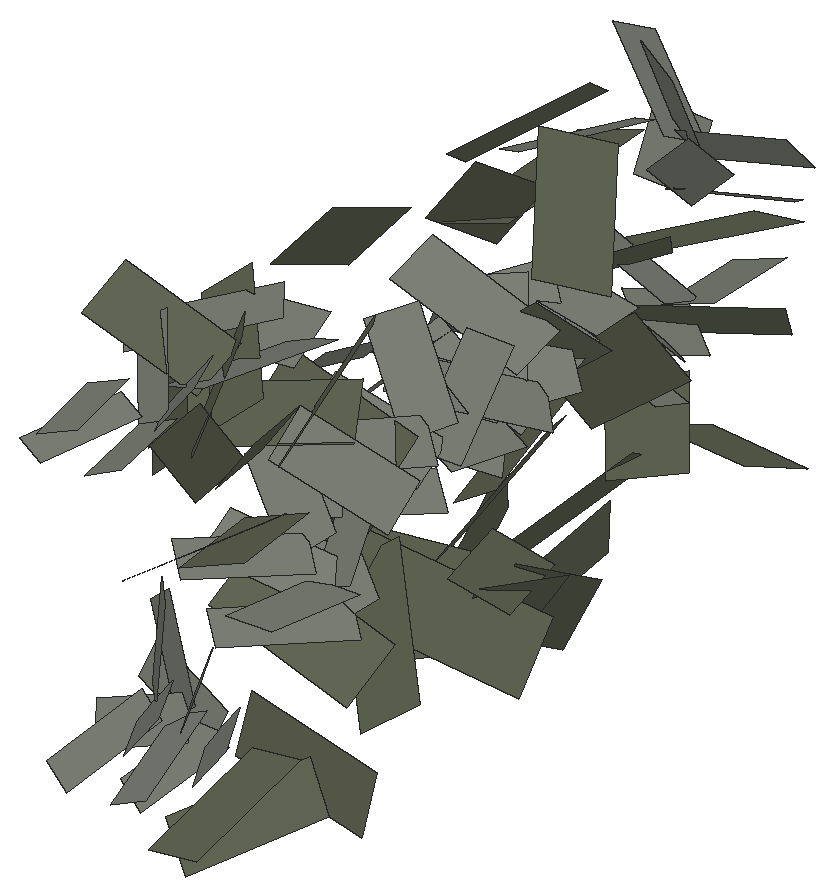
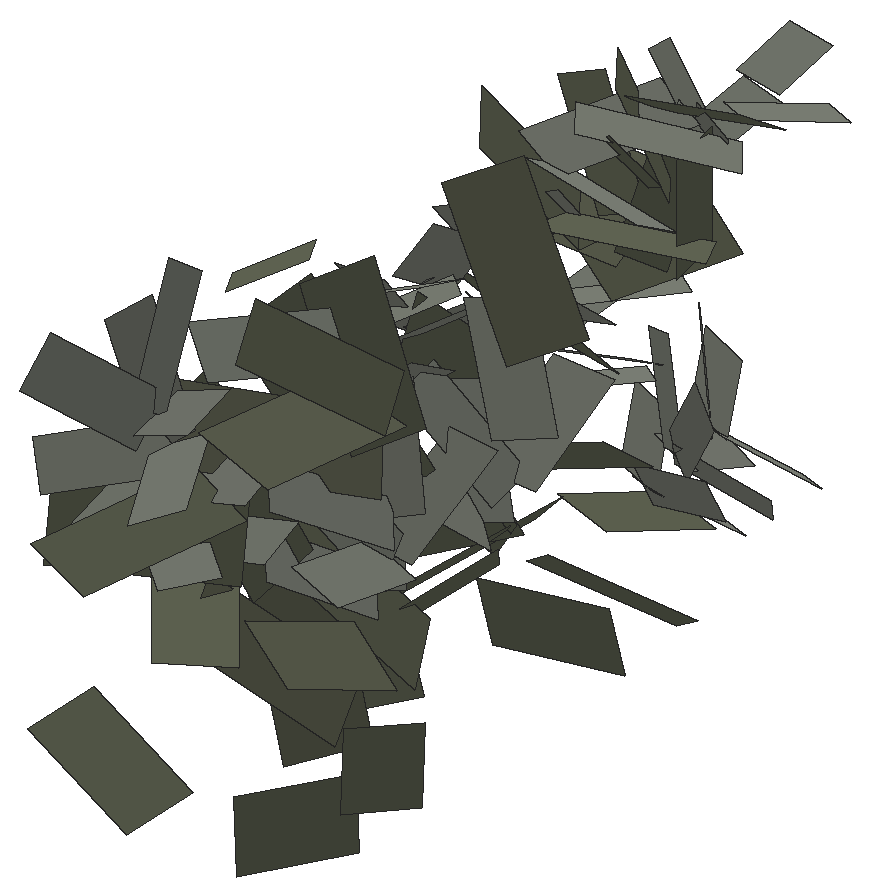
# SketchUp Ruby script. Lengths in inches.
U = 1.inch
M = Sketchup.active_model
def pt(a) = Geom::Point3d.new(a.map { |v| v * U })
def face(e, loops, mat)
  f = e.add_face(loops[0].map { |a| pt(a) })
  loops[1..].each { |l| e.add_face(l.map { |a| pt(a) }).erase! }
  f.material = f.back_material = mat if mat
  f
end
# faces: each face lists its corners as indices into pts; further lists are holes
def faces(e, pts, list, mat = nil) = list.each { |f| face(e, (f[0].is_a?(Array) ? f : [f]).map { |l| l.map { |i| pts[i] } }, mat) }
# xy, xz, yz: faces in a plane at the given z, y or x. An outline is a flat list of corners, or four numbers for a rectangle; further outlines are holes
def ring(l) = l.size == 4 ? [[l[0], l[1]], [l[2], l[1]], [l[2], l[3]], [l[0], l[3]]] : l.each_slice(2).to_a
def flat(e, list, mat, &to3) = list.each { |f| face(e, (f[0].is_a?(Array) ? f : [f]).map { |l| ring(l).map { |u, v| to3.(u, v) } }, mat) }
def xy(e, z, list, mat = nil) = flat(e, list, mat) { |x, y| [x, y, z] }
def xz(e, y, list, mat = nil) = flat(e, list, mat) { |x, z| [x, y, z] }
def yz(e, x, list, mat = nil) = flat(e, list, mat) { |y, z| [x, y, z] }
def lines(e, pts, list) = list.each { |a, b| e.add_line(pt(pts[a]), pt(pts[b])) }
# prism: a flat outline (further loops are holes) pulled along v
def prism(e, loops, v, mat = nil)
  f = face(e, loops, mat); d = Geom::Vector3d.new(v.map { |x| x * U })
  f.pushpull(f.normal.samedirection?(d) ? d.length : -d.length)
end
def box(e, o, s, mat = nil) = prism(e, [[o, [o[0] + s[0], o[1], o[2]], [o[0] + s[0], o[1] + s[1], o[2]], [o[0], o[1] + s[1], o[2]]]], [0, 0, s[2]], mat)
def at(x, y, z, deg = 0) = Geom::Transformation.translation(pt([x, y, z])) * Geom::Transformation.rotation(ORIGIN, Z_AXIS, deg.degrees)
def axes(o, x, y, z) = Geom::Transformation.new([*x, 0, *y, 0, *z, 0, *pt(o).to_a, 1])
def part(name) = M.definitions.add(name)
# library, detail: a bought-in or finely detailed component or shape, given as its bounding box
def library(name, o, s) = part(name).tap { |d| box(d.entities, o, s) }
def detail(e, o, s) = box(e.add_group.entities, o, s)
def put(e, d, t, mat = nil) = e.add_instance(d, t).tap { |i| i.material = mat if mat }
def group(e, t, mat = nil) = e.add_group.tap { |g| g.transformation = t; g.material = mat if mat }.entities
root = M.entities
M.materials.add("viburnumblaasdfas0df1w06d").color = [98, 102, 84]
M.materials.add("viburnumbladsadfasdfad0w122").color = [125, 129, 119]
c1 = part("Component\#315")
p = [[0.25,0,0],[2.05,0.01,0.35],[1.81,4.2,1.66],[0,4.19,1.3125]]
faces(c1.entities,p,[[0,1,2,3]],"viburnumbladsadfasdfad0w122")
c2 = part("viburnumblad2")
put(c2.entities,c1,axes([-19.23,-4.49,-32.18],[83.35428,0,0],[0,79.38502,0],[0,0,83.35428]))
c3 = part("Component\#314")
p = [[0.14,0,0],[2.58,0.05,0.25],[2.44,5.11,2.64],[0,5.05,2.39]]
faces(c3.entities,p,[[0,1,2,3]],"viburnumblaasdfas0df1w06d")
c4 = part("viburnumblad1\#2")
put(c4.entities,c3,axes([-37.25,6.23,19.31],[75.98784,0,0],[0,65.50676,0],[0,0,75.98784]))
put(root,c2,axes([2197.35,270.92,20.94],[0.01264,-0.00008,0.0032],[0.00017,0.01368,-0.00036],[-0.00319,0.00037,0.01263]))
put(root,c4,axes([2198.77,269.1,11.5625],[0.00484,-0.00571,0.01239],[0.00394,0.01587,0.00555],[-0.01361,0.00143,0.00513]))
put(root,c2,axes([2198.79,266.02,22.4375],[-0.0132,-0.00264,-0.00489],[0.00251,-0.01421,0.00089],[-0.00477,0.0001,0.01275]))
put(root,c4,axes([2196.78,266.52,26.34],[-0.0079,-0.01248,0.00117],[0.01398,-0.00821,0.00596],[-0.0035,0.004,0.01323]))
put(root,c2,axes([2199.56,270.78,21.55],[-0.01264,0.00008,-0.0032],[-0.00094,-0.01268,0.00342],[-0.00306,0.00351,0.01217]))
put(root,c4,axes([2198.75,256.2,24.51],[0.00244,-0.01122,0.00057],[0.00459,0.00184,0.0121],[-0.01018,-0.00173,0.00319]))
put(root,c4,axes([2196.55,273.26,27.23],[0.00379,-0.01036,0.00596],[0.01309,0.006,0.00209],[-0.00395,0.00482,0.01088]))
put(root,c4,axes([2201.18,254.32,28.69],[0.00232,0.01057,0.00577],[-0.01348,0.00407,-0.00203],[-0.00316,-0.00514,0.01068]))
put(root,c2,axes([2200.07,251.87,28.74],[-0.00892,0.00552,-0.00065],[-0.0045,-0.00791,-0.00542],[-0.00314,-0.00411,0.00807]))
put(root,c2,axes([2197.68,266.58,23.97],[-0.00718,-0.01175,-0.00394],[0.01087,-0.00815,0.00451],[-0.0058,-0.00063,0.01231]))
put(root,c2,axes([2199.07,252.96,27.46],[0.0088,0.00119,0.00472],[-0.00418,0.00904,0.00526],[-0.00322,-0.0061,0.00681]))
put(root,c4,axes([2197.79,271.04,26.21],[0.01555,-0.00131,0.00405],[0.00291,0.01735,-0.00577],[-0.00307,0.00585,0.01401]))
put(root,c2,axes([2197.32,267.03,20.32],[0.012,-0.00837,0.00311],[0.00592,0.01032,0.00492],[-0.00527,-0.00304,0.01219]))
put(root,c2,axes([2200.45,252.26,17.23],[-0.00876,0.00688,0.00103],[-0.00474,-0.00469,-0.00897],[-0.00509,-0.00746,0.00659]))
put(root,c2,axes([2200.76,253.27,16.05],[-0.0033,0.00751,0.0076],[-0.0089,0.00112,-0.00498],[-0.00448,-0.00819,0.00616]))
put(root,c2,axes([2201.45,257.38,30.71],[-0.00774,0.01238,-0.00167],[-0.01057,-0.00772,-0.00819],[-0.0074,-0.00296,0.01235]))
put(root,c2,axes([2197.1875,267.16,21.98],[0.00305,-0.01398,-0.00068],[0.01153,0.00223,0.00588],[-0.00601,-0.00193,0.01207]))
put(root,c2,axes([2197.29,272.09,22.5],[0.00854,-0.00917,0.00359],[0.00887,0.00923,0.00245],[-0.00426,0.00084,0.01229]))
put(root,c2,axes([2200.6,254.54,15.23],[0.00419,0.0043,0.00836],[-0.00938,0.00585,0.00169],[-0.00405,-0.0083,0.0063]))
put(root,c4,axes([2198.62,270.69,16.26],[0.01227,-0.00323,0.0066],[0.00379,0.01612,0.00085],[-0.00658,0.00088,0.01266]))
put(root,c2,axes([2199.51,254.22,16.22],[0.00908,-0.00221,0.00614],[-0.004,0.00655,0.00828],[-0.00518,-0.00884,0.00448]))
put(root,c2,axes([2199.6,251.82,30.03],[-0.00916,-0.00124,-0.00492],[0.00298,-0.00959,-0.00307],[-0.00406,-0.0039,0.00779]))
put(root,c2,axes([2198.85,271.8,22.94],[-0.00933,-0.00906,-0.00093],[0.0081,-0.00886,0.00508],[-0.00417,0.00306,0.01196]))
put(root,c2,axes([2201.47,257.88,28.64],[0.00099,0.01426,0.00559],[-0.01157,0.00302,-0.00566],[-0.00706,-0.00428,0.01216]))
put(root,c4,axes([2198.25,272.39,25.21],[-0.00969,-0.0086,0.00402],[0.01095,-0.00941,0.00625],[-0.00101,0.00665,0.01178]))
put(root,c4,axes([2199.29,271.49,10.8125],[0.00403,-0.00389,0.01235],[0.00756,0.01368,0.00184],[-0.01119,0.00546,0.00538]))
put(root,c4,axes([2200.93,255.43,26.7],[0.00961,0.00314,0.00694],[-0.00599,0.01265,0.00258],[-0.0056,-0.00466,0.00986]))
put(root,c2,axes([2198.74,267.11,20.93],[-0.00599,-0.01069,-0.00483],[0.01087,-0.00815,0.00451],[-0.00654,-0.00189,0.01181]))
put(root,c2,axes([2199.03,253.58,17.7],[0.00876,-0.00688,-0.00103],[0.00337,0.00275,0.0103],[-0.00608,-0.00838,0.00422]))
put(root,c2,axes([2198.37,272.06,21.01],[-0.00055,-0.01289,0.00188],[0.01116,0.00015,0.00431],[-0.00466,0.00195,0.01201]))
put(root,c2,axes([2198.32,271.62,19.47],[0.00892,-0.00957,0.00375],[0.00799,0.0083,0.0022],[-0.00426,0.00084,0.01229]))
put(root,c2,axes([2201.66,254.26,15.75],[-0.00914,0.00718,0.00108],[-0.00427,-0.00422,-0.00808],[-0.00509,-0.00746,0.00659]))
put(root,c2,axes([2201.97,277.49,28.94],[0.00139,0.01031,-0.00841],[-0.01248,0.00393,0.00276],[0.0046,0.00756,0.01003]))
put(root,c2,axes([2199.63,271.46,19.93],[-0.00812,-0.00859,-0.00204],[0.0081,-0.00886,0.00508],[-0.00515,0.00206,0.01179]))
put(root,c2,axes([2200.54,253.08,28.33],[-0.00798,-0.00075,-0.00527],[0.00298,-0.00959,-0.00307],[-0.00502,-0.00401,0.00721]))
put(root,c4,axes([2204.23,258.62,26.16],[-0.0074,0.01393,0.00333],[-0.01491,-0.00558,-0.00981],[-0.00631,-0.00654,0.01332]))
put(root,c2,axes([2198.41,273.23,29.13],[0.01161,-0.00902,0.00438],[0.00853,0.00943,-0.00297],[-0.0007,0.0056,0.01299]))
put(root,c2,axes([2201.13,276.96,27.46],[0.00973,0.00497,-0.00674],[-0.00836,0.01112,-0.00387],[0.00402,0.00678,0.0108]))
put(root,c4,axes([2200.77,256.64,24.66],[-0.00329,-0.00864,-0.00687],[0.00632,-0.00867,0.00771],[-0.00921,-0.00096,0.00528]))
put(root,c2,axes([2201.15,253.77,17.21],[-0.00908,0.00221,-0.00614],[0.00272,-0.00885,-0.00722],[-0.00599,-0.007,0.00633]))
put(root,c4,axes([2202.68,268.2,14.41],[-0.00681,0.00895,0.00759],[-0.01184,-0.01026,0.00148],[0.00579,-0.00507,0.01117]))
put(root,c4,axes([2200.12,255.04,26.2],[0.00733,-0.00886,0.00054],[0.00689,0.00642,0.00923],[-0.00652,-0.00466,0.00706]))
put(root,c2,axes([2199.67,253.81,28.29],[0.0036,-0.00945,-0.00418],[0.00778,0.00056,0.0052],[-0.00475,-0.00515,0.0067]))
put(root,c4,axes([2199.32,268.54,15.01],[0.00765,-0.01303,0.00422],[0.01267,0.01016,0.00822],[-0.00817,-0.00039,0.01254]))
put(root,c2,axes([2200.23,253.14,18.3],[-0.00409,-0.00375,-0.00971],[0.008,-0.0078,-0.00036],[-0.00665,-0.00708,0.00553]))
put(root,c4,axes([2204.46,259.39,23.27],[0.00378,0.01126,0.01091],[-0.0152,0.00977,-0.00482],[-0.0086,-0.00789,0.01113]))
put(root,c4,axes([2204.01,259.37,11.11],[0.00278,0.00293,0.01264],[-0.01346,0.00734,0.00126],[-0.00579,-0.01128,0.00389]))
put(root,c2,axes([2202.73,258.64,29.79],[-0.01142,0.0037,-0.00741],[-0.00214,-0.01514,-0.00425],[-0.0084,-0.00214,0.01187]))
put(root,c4,axes([2198.46,271.04,23.44],[0.00743,-0.01098,0.00888],[0.01612,0.00899,-0.00172],[-0.00302,0.0089,0.01251]))
put(root,c4,axes([2204.05,257.3,12.875],[-0.00836,0.0066,0.00609],[-0.00962,-0.00288,-0.01008],[-0.00344,-0.01004,0.00615]))
put(root,c2,axes([2202.46,256.5,22.25],[0.00865,0.00796,0.00491],[-0.00918,0.00854,0.00232],[-0.00184,-0.00511,0.01153]))
put(root,c2,axes([2203.73,256.68,20.85],[-0.00016,0.01206,0.00411],[-0.0133,0.00032,-0.00146],[-0.00141,-0.0041,0.01199]))
put(root,c2,axes([2200.19,254.5625,17.43],[0.0033,-0.00751,-0.0076],[0.00833,-0.00317,0.00675],[-0.00669,-0.00765,0.00466]))
put(root,c4,axes([2204.34,258.28,16.42],[0.00263,0.01141,0.00764],[-0.01577,0.00377,-0.0002],[-0.00192,-0.0074,0.01171]))
put(root,c4,axes([2203.01,256.13,23.87],[-0.00905,0.00252,-0.00817],[0.0005,-0.01365,-0.00475],[-0.00803,-0.00297,0.00749]))
put(root,c4,axes([2203.13,265.79,15.03],[-0.01009,0.00576,0.00864],[-0.00958,-0.01423,-0.00203],[0.00708,-0.00619,0.01118]))
put(root,c2,axes([2203.21,265.82,22.78],[0.00269,0.01067,0.0031],[-0.01059,0.00139,0.00439],[0.00368,-0.00386,0.01011]))
put(root,c2,axes([2204.01,256.14,22.52],[-0.00888,0.0091,0.0009],[-0.00895,-0.0084,-0.00345],[-0.00187,-0.00303,0.01224]))
put(root,c4,axes([2199.96,271.49,14.1],[0.00413,-0.01232,0.00597],[0.01417,0.00711,0.00487],[-0.00618,0.00389,0.01229]))
put(root,c2,axes([2204.13,274.625,24.71],[-0.00041,0.01136,-0.00703],[-0.01336,-0.0005,-0.00003],[-0.00029,0.00703,0.01137]))
put(root,c2,axes([2203.77,266.37,21.47],[-0.00563,0.00838,0.00295],[-0.00922,-0.00664,0.00128],[0.00288,-0.0019,0.0109]))
put(root,c4,axes([2200.15,276,24.16],[0.01373,-0.0042,0.00303],[0.00601,0.01319,-0.00893],[-0.00014,0.00827,0.01212]))
put(root,c4,axes([2201.71,260.84,19.45],[0.00372,-0.01109,0.0102],[0.00971,0.0119,0.0094],[-0.01253,0.00356,0.00844]))
put(root,c4,axes([2203.31,256.45,14.86],[-0.01158,0.00263,-0.00305],[0.00041,-0.00999,-0.01013],[-0.00401,-0.00833,0.00806]))
put(root,c2,axes([2201.36,255.22,16.76],[-0.00392,-0.0036,-0.00932],[0.00864,-0.00842,-0.00039],[-0.00665,-0.00708,0.00553]))
put(root,c2,axes([2204.02,261.58,23.2],[-0.00038,0.01114,0.00561],[-0.01176,-0.00241,0.0034],[0.00455,-0.00528,0.01006]))
put(root,c2,axes([2203.17,257.74,19.44],[0.00904,0.00831,0.00513],[-0.00826,0.00768,0.00209],[-0.00184,-0.00511,0.01153]))
put(root,c2,axes([2204.24,265.54,24.03],[-0.00577,0.00885,0.00437],[-0.00922,-0.00664,0.00128],[0.00353,-0.00288,0.01049]))
put(root,c2,axes([2203.42,277.97,28.14],[-0.01295,0.00298,0.00152],[-0.00101,-0.00935,0.0097],[0.0032,0.00918,0.00919]))
put(root,c4,axes([2200.22,269.48,20.91],[-0.01012,-0.01025,0.00891],[0.01634,-0.00922,0.0075],[0.00063,0.01164,0.0125]))
put(root,c2,axes([2204.9,273.17,21.77],[-0.00039,0.0109,-0.00675],[-0.01442,-0.00054,-0.00004],[-0.00029,0.00703,0.01137]))
put(root,c2,axes([2204.95,265.6,26.28],[0,0.01516,0.00154],[-0.01516,-0.00015,0.00148],[0.00149,-0.00153,0.01509]))
put(root,c2,axes([2204.75,257.52,19.71],[-0.00853,0.00873,0.00086],[-0.00967,-0.00907,-0.00372],[-0.00187,-0.00303,0.01224]))
put(root,c4,axes([2205.24,277.81,16.8125],[0.00536,0.01158,-0.00521],[-0.01304,0.00197,-0.00903],[-0.0059,0.00728,0.01011]))
put(root,c4,axes([2203.74,259.76,14.36],[0.01152,0.00345,0.00714],[-0.0073,0.01349,0.00527],[-0.00481,-0.00695,0.01113]))
put(root,c2,axes([2203.85,274.09,22.94],[0.00906,0.00899,-0.00397],[-0.01029,0.00825,-0.00478],[-0.00073,0.006,0.01192]))
put(root,c2,axes([2204.5,262.6,22.03],[-0.00848,0.00652,0.00394],[-0.00785,-0.00971,-0.00119],[0.00311,-0.00363,0.01115]))
put(root,c2,axes([2202.95,265.99,24.48],[0.00958,0.00624,0.00001],[-0.00544,0.00834,0.00562],[0.00306,-0.00472,0.00995]))
put(root,c4,axes([2204.25,271.86,18.51],[0.01166,0.00889,0.00003],[-0.00952,0.01251,-0.00648],[-0.00341,0.00442,0.01356]))
put(root,c2,axes([2203.61,261.32,24.9375],[0.00829,0.0091,0.00248],[-0.00839,0.00593,0.00669],[0.00415,-0.0063,0.00965]))
put(root,c4,axes([2201.64,256.24,25.51],[-0.001,-0.01064,-0.00433],[0.01169,-0.00333,0.00541],[-0.00539,-0.00308,0.00855]))
put(root,c4,axes([2201.95,257.23,24.94],[0.00803,-0.00983,0.00384],[0.00868,0.0101,0.00771],[-0.00745,-0.00186,0.01082]))
put(root,c2,axes([2205.34,274.15,23.19],[-0.00964,0.00707,-0.00598],[-0.00922,-0.00808,0.00531],[-0.0008,0.00796,0.01071]))
put(root,c2,axes([2202.61,257.68,20.89],[0.0124,-0.0008,0.00284],[-0.00048,0.01054,0.00506],[-0.0029,-0.00547,0.01114]))
put(root,c4,axes([2202.19,270.84,11.95],[-0.01097,-0.01069,0.00215],[0.01213,-0.01096,0.00739],[-0.00308,0.00597,0.01392]))
put(root,c2,axes([2204.29,266.25,24.39],[0.01077,0.01069,0.00135],[-0.01074,0.01048,0.00267],[0.00094,-0.00284,0.01494]))
put(root,c4,axes([2203.45,256.45,23.95],[-0.01126,-0.00328,-0.00424],[0.0051,-0.0131,-0.00341],[-0.00278,-0.00386,0.0103]))
put(root,c2,axes([2205.125,261.29,24.55],[-0.00883,0.00666,0.00546],[-0.00785,-0.00971,-0.00119],[0.00409,-0.00438,0.01062]))
put(root,c4,axes([2201.96,268.95,12.97],[-0.00857,-0.01458,-0.00131],[0.01562,-0.00975,0.00697],[-0.00558,0.00226,0.01502]))
put(root,c4,axes([2206.37,264.7,14.89],[0.00192,0.00886,0.01301],[-0.01818,-0.00012,0.00276],[0.00142,-0.01315,0.00875]))
put(root,c2,axes([2204.56,266.7,22.76],[-0.01085,0.00184,0.00308],[-0.00218,-0.01013,-0.00164],[0.00269,-0.00234,0.01086]))
put(root,c4,axes([2201.47,273.13,19.36],[-0.01045,-0.00476,0.01095],[0.01292,-0.01059,0.00773],[0.00429,0.01208,0.00936]))
put(root,c2,axes([2201.45,278.26,26.41],[0.00854,-0.00981,0.00509],[0.00939,0.0055,-0.00515],[0.00179,0.0073,0.01107]))
put(root,c2,axes([2205.48,269.05,26.37],[0.00259,0.01229,-0.00001],[-0.01185,0.00249,-0.00335],[-0.00327,0.0007,0.01211]))
put(root,c2,axes([2202.84,277.87,26.44],[-0.00947,-0.00564,0.00547],[0.00849,-0.00835,0.00609],[0.00092,0.00846,0.01032]))
put(root,c4,axes([2200.5,275.35,21.53],[0.00481,-0.00968,0.00992],[0.01607,0.00349,-0.00438],[0.00046,0.01061,0.01012]))
put(root,c4,axes([2204.73,267.1875,28.21],[0.00918,0.0099,-0.00625],[-0.01245,0.01197,0.0007],[0.0045,0.00408,0.01216]))
put(root,c2,axes([2206.22,265.95,24.4],[-0.01077,0.01075,0.00083],[-0.01084,-0.01091,0.00051],[0.00094,-0.00022,0.01521]))
put(root,c2,axes([2204.78,257.48,21.42],[-0.0124,0.0008,-0.00284],[-0.0002,-0.01247,-0.00265],[-0.00294,-0.00253,0.01214]))
put(root,c2,axes([2203.13,275.7,23.875],[0.01322,0.00136,0.00142],[-0.00064,0.01212,-0.00561],[-0.00186,0.00548,0.01205]))
put(root,c2,axes([2202.67,267.06,23.34],[0.01085,-0.00184,-0.00308],[0.00296,0.01015,0.00436],[0.00203,-0.00494,0.01011]))
put(root,c2,axes([2203.06,262.6,23.95],[0.01211,0.00173,-0.00211],[0,0.01038,0.00684],[0.00312,-0.00685,0.00964]))
put(root,c4,axes([2203.71,268.75,16.93],[-0.01133,-0.00353,0.00405],[0.00312,-0.01382,-0.0033],[0.00465,-0.0017,0.01152]))
put(root,c2,axes([2206.07,257.25,24.06],[0.00252,0.00942,0.00914],[-0.01307,0.00092,0.00265],[0.00124,-0.00944,0.00938]))
put(root,c2,axes([2202.26,279.27,27.42],[-0.00139,-0.01031,0.00841],[0.01214,-0.00182,-0.00024],[0.00145,0.00829,0.0104]))
